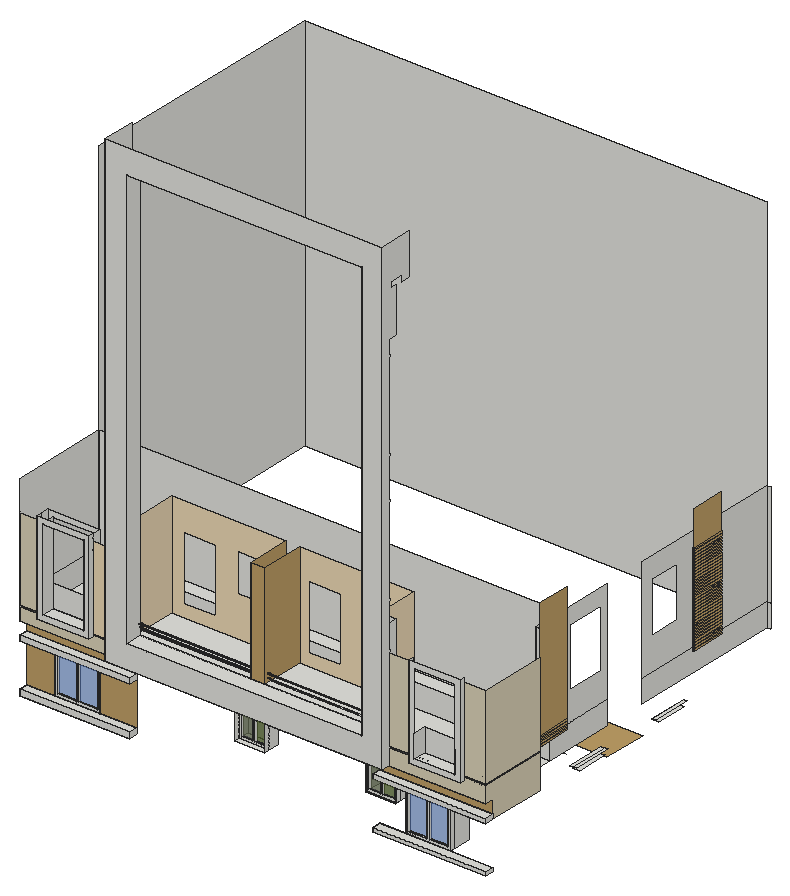
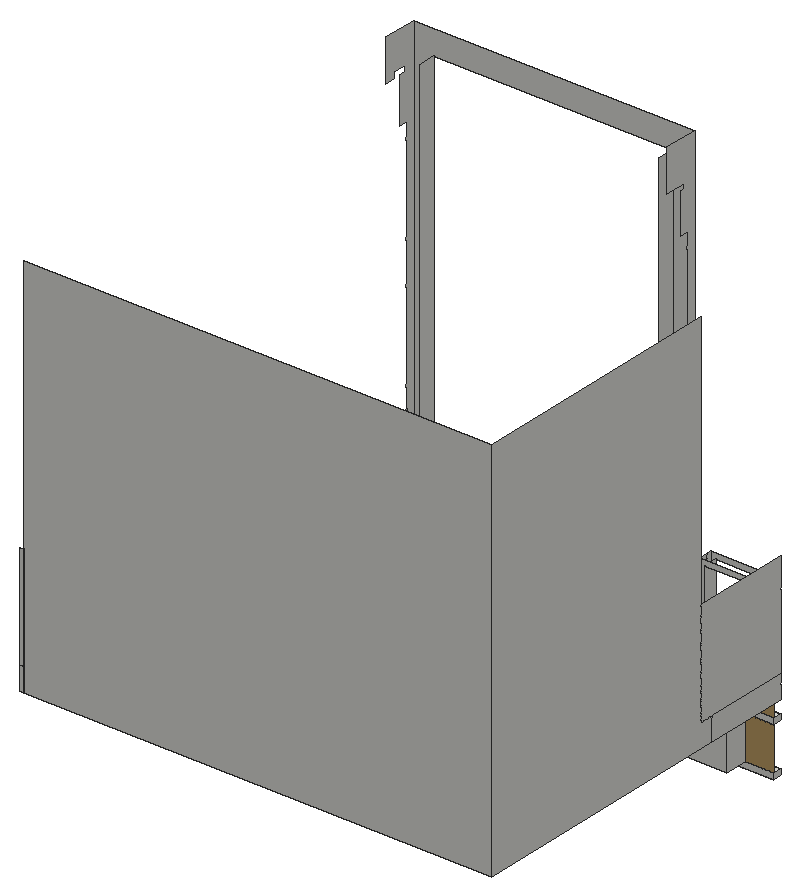
# SketchUp Ruby script. Lengths in inches.
U = 1.inch
M = Sketchup.active_model
def pt(a) = Geom::Point3d.new(a.map { |v| v * U })
def face(e, loops, mat)
  f = e.add_face(loops[0].map { |a| pt(a) })
  loops[1..].each { |l| e.add_face(l.map { |a| pt(a) }).erase! }
  f.material = f.back_material = mat if mat
  f
end
# faces: each face lists its corners as indices into pts; further lists are holes
def faces(e, pts, list, mat = nil) = list.each { |f| face(e, (f[0].is_a?(Array) ? f : [f]).map { |l| l.map { |i| pts[i] } }, mat) }
# xy, xz, yz: faces in a plane at the given z, y or x. An outline is a flat list of corners, or four numbers for a rectangle; further outlines are holes
def ring(l) = l.size == 4 ? [[l[0], l[1]], [l[2], l[1]], [l[2], l[3]], [l[0], l[3]]] : l.each_slice(2).to_a
def flat(e, list, mat, &to3) = list.each { |f| face(e, (f[0].is_a?(Array) ? f : [f]).map { |l| ring(l).map { |u, v| to3.(u, v) } }, mat) }
def xy(e, z, list, mat = nil) = flat(e, list, mat) { |x, y| [x, y, z] }
def xz(e, y, list, mat = nil) = flat(e, list, mat) { |x, z| [x, y, z] }
def yz(e, x, list, mat = nil) = flat(e, list, mat) { |y, z| [x, y, z] }
def lines(e, pts, list) = list.each { |a, b| e.add_line(pt(pts[a]), pt(pts[b])) }
# prism: a flat outline (further loops are holes) pulled along v
def prism(e, loops, v, mat = nil)
  f = face(e, loops, mat); d = Geom::Vector3d.new(v.map { |x| x * U })
  f.pushpull(f.normal.samedirection?(d) ? d.length : -d.length)
end
def box(e, o, s, mat = nil) = prism(e, [[o, [o[0] + s[0], o[1], o[2]], [o[0] + s[0], o[1] + s[1], o[2]], [o[0], o[1] + s[1], o[2]]]], [0, 0, s[2]], mat)
def at(x, y, z, deg = 0) = Geom::Transformation.translation(pt([x, y, z])) * Geom::Transformation.rotation(ORIGIN, Z_AXIS, deg.degrees)
def axes(o, x, y, z) = Geom::Transformation.new([*x, 0, *y, 0, *z, 0, *pt(o).to_a, 1])
def part(name) = M.definitions.add(name)
# library, detail: a bought-in or finely detailed component or shape, given as its bounding box
def library(name, o, s) = part(name).tap { |d| box(d.entities, o, s) }
def detail(e, o, s) = box(e.add_group.entities, o, s)
def put(e, d, t, mat = nil) = e.add_instance(d, t).tap { |i| i.material = mat if mat }
def group(e, t, mat = nil) = e.add_group.tap { |g| g.transformation = t; g.material = mat if mat }.entities
root = M.entities
M.materials.add("Generic").color = [191, 159, 103]
M.materials.add("Generic\#2").color = [235, 215, 180]
M.materials.add("Generic\#3").color = [218, 209, 183]
M.materials.add("[Color M06]").color = [86, 86, 86]
M.materials.add("[Translucent Glass Blue]").color = [100, 149, 237]
M.materials["[Translucent Glass Blue]"].alpha = 0.5
M.materials.add("[Translucent Glass Dark Green]").color = [62, 91, 5]
M.materials["[Translucent Glass Dark Green]"].alpha = 0.5
M.materials.add("[Translucent Glass Gray]").color = [128, 128, 128]
M.materials["[Translucent Glass Gray]"].alpha = 0.5
c1 = part("Group\#3")
xy(c1.entities,0,[[0,0,51.8125,6]])
xy(c1.entities,4.04,[[4.04,0,23.89,3],[27.93,0,47.77,3]])
xy(c1.entities,53.71,[[4.04,0,23.89,3],[27.93,0,47.77,3]])
xy(c1.entities,57.75,[[0,0,51.8125,6]])
xz(c1.entities,0,[[[0,0,51.8125,57.75],[4.04,4.04,23.89,53.71],[27.93,4.04,47.77,53.71]]])
xz(c1.entities,3,[[4.04,4.04,23.89,53.71],[27.93,4.04,47.77,53.71]],"[Translucent Glass Dark Green]")
xz(c1.entities,6,[[0,0,51.8125,57.75]],"[Translucent Glass Gray]")
yz(c1.entities,0,[[0,0,6,57.75]])
yz(c1.entities,4.04,[[0,4.04,3,53.71]])
yz(c1.entities,23.89,[[0,4.04,3,53.71]])
yz(c1.entities,27.93,[[0,4.04,3,53.71]])
yz(c1.entities,47.77,[[0,4.04,3,53.71]])
yz(c1.entities,51.8125,[[0,0,6,57.75]])
c2 = part("Group\#2")
xy(c2.entities,0,[[0,0,77.5625,6]])
xy(c2.entities,4.2,[[4.2,0,36.68,3],[40.88,0,73.36,3]])
xy(c2.entities,70.05,[[4.2,0,36.68,3],[40.88,0,73.36,3]])
xy(c2.entities,74.25,[[0,0,77.5625,6]])
xz(c2.entities,0,[[[0,0,77.5625,74.25],[40.88,4.2,73.36,70.05],[4.2,4.2,36.68,70.05]]])
xz(c2.entities,3,[[4.2,4.2,36.68,70.05],[40.88,4.2,73.36,70.05]],"[Translucent Glass Blue]")
xz(c2.entities,6,[[0,0,77.5625,74.25]])
yz(c2.entities,0,[[0,0,6,74.25]])
yz(c2.entities,4.2,[[0,4.2,3,70.05]])
yz(c2.entities,36.68,[[0,4.2,3,70.05]])
yz(c2.entities,40.88,[[0,4.2,3,70.05]])
yz(c2.entities,73.36,[[0,4.2,3,70.05]])
yz(c2.entities,77.5625,[[0,0,6,74.25]])
c3 = part("Group\#5")
xy(c3.entities,0,[[0,0,1,57.75]])
xy(c3.entities,2.57,[[0,0,1,57.75]])
xz(c3.entities,0,[[0,0,1,2.57]])
xz(c3.entities,57.75,[[0,0,1,2.57]])
yz(c3.entities,1,[[0,0,57.75,2.57]])
c4 = part("Group\#6")
put(c4.entities,c3,at(0,0,4.75))
put(c4.entities,c3,at(0,0,0))
put(c4.entities,c3,at(0,0,19))
put(c4.entities,c3,at(0,0,28.5))
put(c4.entities,c3,at(0,0,133))
put(c4.entities,c3,at(0,0,152))
put(c4.entities,c3,at(0,0,128.25))
put(c4.entities,c3,at(0,0,9.5))
put(c4.entities,c3,at(0,0,123.5))
put(c4.entities,c3,at(0,0,114))
put(c4.entities,c3,at(0,0,147.25))
put(c4.entities,c3,at(0,0,118.75))
put(c4.entities,c3,at(0,0,142.5))
put(c4.entities,c3,at(0,0,109.25))
put(c4.entities,c3,at(0,0,137.75))
put(c4.entities,c3,at(0,0,104.5))
put(c4.entities,c3,at(0,0,99.75))
put(c4.entities,c3,at(0,0,95))
put(c4.entities,c3,at(0,0,85.5))
put(c4.entities,c3,at(0,0,80.75))
put(c4.entities,c3,at(0,0,90.25))
put(c4.entities,c3,at(0,0,76))
put(c4.entities,c3,at(0,0,71.25))
put(c4.entities,c3,at(0,0,38))
put(c4.entities,c3,at(0,0,14.25))
put(c4.entities,c3,at(0,0,33.25))
put(c4.entities,c3,at(0,0,57))
put(c4.entities,c3,at(0,0,23.75))
put(c4.entities,c3,at(0,0,61.75))
put(c4.entities,c3,at(0,0,156.75))
put(c4.entities,c3,at(0,0,47.5))
put(c4.entities,c3,at(0,0,52.25))
put(c4.entities,c3,at(0,0,42.75))
put(c4.entities,c3,at(0,0,66.5))
xy(root,284.38,[[4.1875,68.4375,193.83,83.8125]])
xy(root,286.25,[[310.76,150.125,362.58,158.75],[536.08,150.125,587.89,158.75],[310.76,158.75,362.58,177.1875],[536.08,158.75,587.89,210.9375]])
xy(root,287.13,[[613.73,68.4375,809.375,83.8125]])
xy(root,294.19,[[4.1875,68.4375,193.83,83.8125],[613.73,68.4375,809.375,83.8125],[53.01,83.8125,130.57,121.875],[658.76,83.8125,736.32,121.875]])
xy(root,344,[[310.76,150.125,362.58,158.75],[536.08,150.125,587.89,158.75],[310.76,158.75,362.58,177.1875],[536.08,158.75,587.89,210.9375]])
xy(root,344.97,[[214.375,158.75,270.0625,214.75],[439.6875,158.75,495.375,214.75]])
xy(root,348.04,[[306.72,150.125,366.62,158.75],[532.04,150.125,591.93,158.75]])
xy(root,350.51,[[710.73,338.625,802.875,414.4375]],"Generic")
xy(root,367.13,[[802.875,263.64,815.3125,317.96],[802.875,434.88,815.3125,489.19]])
xy(root,368.44,[[4.1875,68.4375,193.83,83.8125],[53.01,83.8125,130.57,121.875],[658.76,83.8125,736.32,121.875]])
xy(root,368.76,[[613.23,68.4375,809.375,83.8125]])
xy(root,373.53,[[802.875,257.24,809.375,324.36],[809.375,257.24,815.3125,324.36],[809.375,428.47,815.3125,495.59]])
xy(root,376.76,[[613.23,68.4375,809.375,83.8125]])
xy(root,378.07,[[4.1875,68.4375,193.83,83.8125]])
xy(root,399.75,[[162.33,54.3125,641.55,83.8125],[4.1875,68.5,162.33,83.8125],[641.55,68.5,809.375,83.8125],[4.1875,83.8125,4.1875,214.75,802.875,214.75,802.875,83.8125,613.23,83.8125,613.23,158.75,415.53,158.75,415.53,83.8125,391.53,83.8125,391.53,158.75,193.83,158.75,193.83,83.8125],[193.83,83.8125,391.53,158.75],
  [415.53,83.8125,613.23,158.75]])
xy(root,419.29,[[40.68,60.5625,129.91,68.5],[40.68,68.5,129.91,83.8125]])
xy(root,421.51,[[4.1875,68.5,40.68,69.9375],[129.91,68.5,162.33,69.9375]])
xy(root,421.94,[[682.51,60.5625,771.75,68.5]])
xy(root,424.51,[[4.1875,68.5,40.68,69.9375],[129.91,68.5,162.33,69.9375]])
xy(root,427.125,[[641.55,68.5,682.51,69.9375],[771.75,68.5,802.875,69.9375],[802.875,68.5,809.375,69.9375],[807.9375,69.9375,809.375,185.01]])
xy(root,428.19,[[49.58,60.5625,121.01,83.8125]])
xy(root,430.125,[[641.55,68.5,682.51,69.9375],[771.75,68.5,809.375,69.9375],[807.9375,69.9375,809.375,185.01]])
xy(root,430.84,[[691.41,60.5625,762.85,83.8125]])
xy(root,439.5,[[200.02,54.3125,607.05,83.8125],[193.83,83.8125,391.53,158.75],[415.53,83.8125,613.23,158.75],[802.875,185.01,809.375,242.76],[4.1875,214.75,802.875,239.73]])
xz(root,54.3125,[[[162.33,399.75,641.55,1207.3125],[200.02,439.5,607.05,1165.125]]])
xz(root,60.5625,[[[40.68,419.29,129.91,578.68],[49.58,428.19,121.01,569.78]],[[682.51,421.94,771.75,581.34],[691.41,430.84,762.85,572.44]]])
xz(root,68.4375,[[4.1875,284.38,193.83,294.19],[613.73,287.13,809.375,294.19],[4.1875,368.44,193.83,378.07],[613.23,368.76,809.375,376.76]])
xz(root,68.5,[[129.35,421.51,129.91,424.51],[682.51,427.125,771.75,430.125]])
xz(root,68.5,[[129.91,424.51,162.33,567.15]],"Generic\#2")
xz(root,68.5,[[4.1875,399.75,162.33,399.75,162.33,421.51,129.91,421.51,129.91,419.29,40.68,419.29,40.68,421.51,4.1875,421.51],[641.55,399.75,809.375,399.75,809.375,427.125,771.75,427.125,771.75,421.94,682.51,421.94,682.51,427.125,641.55,427.125],[4.1875,424.51,40.68,567.15],[641.55,430.125,682.51,574.59],[771.75,430.125,809.375,574.59]],"Generic\#3")
xz(root,69.9375,[[4.1875,421.51,40.68,424.51],[129.91,421.51,162.33,424.51],[641.55,427.125,682.51,430.125],[771.75,427.125,807.9375,430.125]],"[Color M06]")
xz(root,83.8125,[[4.1875,284.38,193.83,294.19],[613.73,287.13,809.375,294.19],[4.1875,368.44,193.83,378.07],[613.23,368.76,809.375,376.76],[162.33,399.75,607.05,439.5],
  [607.05,399.75,641.55,439.5],[[40.68,419.29,129.91,578.68],[49.58,428.19,121.01,569.78]],[49.58,428.19,121.01,467.03],[691.41,430.84,762.85,469.69],[162.33,439.5,193.83,619.5],
  [193.83,439.5,200.02,619.5],[607.05,439.5,613.23,619.5],[613.23,439.5,641.55,619.5]])
xz(root,83.8125,[[4.1875,294.19,53.01,368.44],[130.57,294.19,193.83,368.44],[613.23,376.76,809.375,399.75],[4.1875,378.07,193.83,399.75],[391.53,439.5,415.53,619.5]],"Generic")
xz(root,121.875,[[53.01,294.19,130.57,368.44],[658.76,294.19,736.32,368.44]])
xz(root,158.75,[[[193.83,439.5,391.53,619.5],[215.38,461.3125,271.07,571.5625],[307.73,508.8,367.625,574.63]],[[415.53,439.5,613.23,619.5],[431.19,461.3125,486.88,571.5625],[523.54,508.8,583.4375,574.63]]],"Generic\#2")
xz(root,177.1875,[[310.76,286.25,362.58,344]])
xz(root,185.01,[[807.9375,427.125,809.375,430.125],[802.875,439.5,802.875,619.5,809.375,619.5,809.375,577.59,807.9375,577.59,807.9375,574.59,809.375,574.59,809.375,439.5]])
xz(root,210.9375,[[536.08,286.25,587.89,344]])
xz(root,214.75,[[4.1875,399.75,802.875,439.5]])
xz(root,239.73,[[4.1875,439.5,802.875,619.5]])
xz(root,242.76,[[802.875,439.5,809.375,619.5]])
xz(root,683.8125,[[4.1875,399.75,802.875,1059],[802.875,399.75,809.375,439.5],[802.875,439.5,809.375,619.5]])
yz(root,4.1875,[[68.4375,284.38,83.8125,294.19],[68.4375,368.44,83.8125,378.07],[68.5,399.75,68.5,421.51,69.9375,421.51,69.9375,424.51,68.5,424.51,68.5,439.5,214.75,439.5,214.75,399.75],[214.75,399.75,214.75,439.5,239.73,439.5,239.73,1059,683.8125,1059,683.8125,399.75],[68.5,439.5,68.5,567.15,69.9375,567.15,69.9375,570.15,68.5,570.15,68.5,619.5,239.73,619.5,239.73,439.5]])
yz(root,40.68,[[60.5625,419.29,68.5,419.29,68.5,421.51,69.9375,421.51,69.9375,424.51,68.5,424.51,68.5,567.15,69.9375,567.15,69.9375,570.15,68.5,570.15,68.5,578.68,60.5625,578.68],[68.5,419.29,83.8125,419.29,83.8125,578.68,68.5,578.68,68.5,570.15,69.9375,570.15,69.9375,567.15,68.5,567.15,68.5,424.51,69.9375,424.51,69.9375,421.51,68.5,421.51]])
yz(root,49.58,[[60.5625,428.19,83.8125,569.78]])
yz(root,53.01,[[83.8125,294.19,121.875,368.44]])
yz(root,121.01,[[60.5625,428.19,83.8125,569.78]])
yz(root,129.91,[[60.5625,419.29,68.5,578.68],[68.5,419.29,68.5,421.51,69.9375,421.51,69.9375,424.51,68.5,424.51,68.5,567.15,69.9375,567.15,69.9375,570.15,68.5,570.15,68.5,578.68,83.8125,578.68,83.8125,419.29],[68.5,421.51,69.9375,424.51]])
yz(root,130.57,[[83.8125,294.19,121.875,368.44]])
yz(root,162.33,[[54.3125,399.75,54.3125,1207.3125,112.625,1207.3125,112.625,1136.625,77.8125,1136.625,77.8125,1128.4375,83.8125,1128.4375,83.8125,1059,68.5,1059,68.5,1036.33,71.375,1036.33,71.375,1033.33,68.5,1033.33,68.5,882,69.9375,882,69.9375,879,68.5,879,68.5,806.75,69.9375,806.75,69.9375,803.75,68.5,803.75,68.5,658.14,69.9375,658.14,69.9375,655.14,68.5,655.14,68.5,570.15,69.9375,570.15,69.9375,567.15,68.5,567.15,68.5,424.51,69.9375,424.51,69.9375,421.51,68.5,421.51,68.5,399.75],[68.5,399.75,68.5,421.51,69.9375,421.51,69.9375,424.51,68.5,424.51,68.5,439.5,83.8125,439.5,83.8125,399.75],[68.5,439.5,68.5,567.15,69.9375,567.15,69.9375,570.15,68.5,570.15,68.5,619.5,83.8125,619.5,83.8125,439.5]])
yz(root,193.83,[[68.4375,284.38,83.8125,294.19],[68.4375,368.44,83.8125,378.07]])
yz(root,193.83,[[[83.8125,439.5,158.75,619.5],[90.04,472.27,89.73,472.3125,89.44,472.43,89.2,472.62,89.01,472.86,88.89,473.15,88.85,473.46,88.89,473.77,89.01,474.05,89.2,474.3,89.44,474.49,89.73,474.61,90.04,474.65,90.35,474.61,90.63,474.49,90.88,474.3,91.07,474.05,91.18,473.77,91.23,473.46,91.18,473.15,91.07,472.86,90.88,472.62,90.63,472.43,90.35,472.3125],[90.04,465.71,89.73,465.75,89.44,465.87,89.2,466.06,89.01,466.3,88.89,466.59,88.85,466.9,88.89,467.2,89.01,467.49,89.2,467.74,89.44,467.92,89.73,468.04,90.04,468.08,90.35,468.04,90.63,467.92,90.88,467.74,91.07,467.49,91.18,467.2,91.23,466.9,91.18,466.59,91.07,466.3,90.88,466.06,90.63,465.87,90.35,465.75],[90.04,458.71,89.73,458.75,89.44,458.87,89.2,459.06,89.01,459.3,88.89,459.59,88.85,459.9,88.89,460.2,89.01,460.49,89.2,460.74,89.44,460.92,89.73,461.04,90.04,461.08,90.35,461.04,90.63,460.92,90.88,460.74,91.07,460.49,91.18,460.2,91.23,459.9,91.18,459.59,91.07,459.3,90.88,459.06,90.63,458.87,90.35,458.75],[90.04,451.71,89.73,451.75,89.44,451.87,89.2,452.06,89.01,452.3,88.89,452.59,88.85,452.9,88.89,453.2,89.01,453.49,89.2,453.74,89.44,453.92,89.73,454.04,90.04,454.08,90.35,454.04,90.63,453.92,90.88,453.74,91.07,453.49,91.18,453.2,91.23,452.9,91.18,452.59,91.07,452.3,90.88,452.06,90.63,451.87,90.35,451.75],[90.04,445.02,89.73,445.0625,89.44,445.18,89.2,445.37,89.01,445.61,88.89,445.9,88.85,446.21,88.89,446.52,89.01,446.8,89.2,447.05,89.44,447.24,89.73,447.36,90.04,447.4,90.35,447.36,90.63,447.24,90.88,447.05,91.07,446.8,91.18,446.52,91.23,446.21,91.18,445.9,91.07,445.61,90.88,445.37,90.63,445.18,90.35,445.0625]]],"Generic\#2")
yz(root,200.02,[[54.3125,439.5,83.8125,1165.125]])
yz(root,310.76,[[150.125,286.25,158.75,344],[158.75,286.25,177.1875,344]])
yz(root,362.58,[[150.125,286.25,158.75,344],[158.75,286.25,177.1875,344]])
yz(root,391.53,[[[83.8125,439.5,158.75,619.5],[90.04,445.02,90.35,445.0625,90.63,445.18,90.88,445.37,91.07,445.61,91.18,445.9,91.23,446.21,91.18,446.52,91.07,446.8,90.88,447.05,90.63,447.24,90.35,447.36,90.04,447.4,89.73,447.36,89.44,447.24,89.2,447.05,89.01,446.8,88.89,446.52,88.85,446.21,88.89,445.9,89.01,445.61,89.2,445.37,89.44,445.18,89.73,445.0625],[90.04,451.71,90.35,451.75,90.63,451.87,90.88,452.06,91.07,452.3,91.18,452.59,91.23,452.9,91.18,453.2,91.07,453.49,90.88,453.74,90.63,453.92,90.35,454.04,90.04,454.08,89.73,454.04,89.44,453.92,89.2,453.74,89.01,453.49,88.89,453.2,88.85,452.9,88.89,452.59,89.01,452.3,89.2,452.06,89.44,451.87,89.73,451.75],[90.04,458.71,90.35,458.75,90.63,458.87,90.88,459.06,91.07,459.3,91.18,459.59,91.23,459.9,91.18,460.2,91.07,460.49,90.88,460.74,90.63,460.92,90.35,461.04,90.04,461.08,89.73,461.04,89.44,460.92,89.2,460.74,89.01,460.49,88.89,460.2,88.85,459.9,88.89,459.59,89.01,459.3,89.2,459.06,89.44,458.87,89.73,458.75],[90.04,465.71,90.35,465.75,90.63,465.87,90.88,466.06,91.07,466.3,91.18,466.59,91.23,466.9,91.18,467.2,91.07,467.49,90.88,467.74,90.63,467.92,90.35,468.04,90.04,468.08,89.73,468.04,89.44,467.92,89.2,467.74,89.01,467.49,88.89,467.2,88.85,466.9,88.89,466.59,89.01,466.3,89.2,466.06,89.44,465.87,89.73,465.75],[90.04,472.27,90.35,472.3125,90.63,472.43,90.88,472.62,91.07,472.86,91.18,473.15,91.23,473.46,91.18,473.77,91.07,474.05,90.88,474.3,90.63,474.49,90.35,474.61,90.04,474.65,89.73,474.61,89.44,474.49,89.2,474.3,89.01,474.05,88.89,473.77,88.85,473.46,88.89,473.15,89.01,472.86,89.2,472.62,89.44,472.43,89.73,472.3125]]],"Generic")
yz(root,415.53,[[[83.8125,439.5,158.75,619.5],[89.21,476.09,89.0625,476.11,88.93,476.16,88.8125,476.25,88.72,476.37,88.67,476.5,88.65,476.65,88.67,476.79,88.72,476.93,88.8125,477.05,88.93,477.14,89.0625,477.19,89.21,477.21,89.36,477.19,89.49,477.14,89.61,477.05,89.7,476.93,89.75,476.79,89.77,476.65,89.75,476.5,89.7,476.37,89.61,476.25,89.49,476.16,89.36,476.11],[89.21,468.65,89.0625,468.67,88.93,468.72,88.8125,468.8125,88.72,468.93,88.67,469.07,88.65,469.21,88.67,469.36,88.72,469.49,88.8125,469.61,88.93,469.7,89.0625,469.76,89.21,469.77,89.36,469.76,89.49,469.7,89.61,469.61,89.7,469.49,89.75,469.36,89.77,469.21,89.75,469.07,89.7,468.93,89.61,468.8125,89.49,468.72,89.36,468.67],[89.21,461.15,89.0625,461.17,88.93,461.22,88.8125,461.3125,88.72,461.43,88.67,461.57,88.65,461.71,88.67,461.86,88.72,461.99,88.8125,462.11,88.93,462.2,89.0625,462.26,89.21,462.27,89.36,462.26,89.49,462.2,89.61,462.11,89.7,461.99,89.75,461.86,89.77,461.71,89.75,461.57,89.7,461.43,89.61,461.3125,89.49,461.22,89.36,461.17],[89.21,453.65,89.0625,453.67,88.93,453.72,88.8125,453.8125,88.72,453.93,88.67,454.07,88.65,454.21,88.67,454.36,88.72,454.49,88.8125,454.61,88.93,454.7,89.0625,454.76,89.21,454.77,89.36,454.76,89.49,454.7,89.61,454.61,89.7,454.49,89.75,454.36,89.77,454.21,89.75,454.07,89.7,453.93,89.61,453.8125,89.49,453.72,89.36,453.67],[89.21,446.27,89.0625,446.29,88.93,446.35,88.8125,446.4375,88.72,446.56,88.67,446.69,88.65,446.84,88.67,446.98,88.72,447.12,88.8125,447.23,88.93,447.32,89.0625,447.38,89.21,447.4,89.36,447.38,89.49,447.32,89.61,447.23,89.7,447.12,89.75,446.98,89.77,446.84,89.75,446.69,89.7,446.56,89.61,446.4375,89.49,446.35,89.36,446.29]]],"Generic")
yz(root,536.08,[[150.125,286.25,158.75,344],[158.75,286.25,210.9375,344]])
yz(root,587.89,[[150.125,286.25,158.75,344],[158.75,286.25,210.9375,344]])
yz(root,607.05,[[54.3125,439.5,83.8125,1165.125]])
yz(root,613.23,[[68.4375,368.76,83.8125,376.76]])
yz(root,613.23,[[[83.8125,439.5,158.75,619.5],[89.21,446.27,89.36,446.29,89.49,446.35,89.61,446.4375,89.7,446.56,89.75,446.69,89.77,446.84,89.75,446.98,89.7,447.12,89.61,447.23,89.49,447.32,89.36,447.38,89.21,447.4,89.0625,447.38,88.93,447.32,88.8125,447.23,88.72,447.12,88.67,446.98,88.65,446.84,88.67,446.69,88.72,446.56,88.8125,446.4375,88.93,446.35,89.0625,446.29],[89.21,453.65,89.36,453.67,89.49,453.72,89.61,453.8125,89.7,453.93,89.75,454.07,89.77,454.21,89.75,454.36,89.7,454.49,89.61,454.61,89.49,454.7,89.36,454.76,89.21,454.77,89.0625,454.76,88.93,454.7,88.8125,454.61,88.72,454.49,88.67,454.36,88.65,454.21,88.67,454.07,88.72,453.93,88.8125,453.8125,88.93,453.72,89.0625,453.67],[89.21,461.15,89.36,461.17,89.49,461.22,89.61,461.3125,89.7,461.43,89.75,461.57,89.77,461.71,89.75,461.86,89.7,461.99,89.61,462.11,89.49,462.2,89.36,462.26,89.21,462.27,89.0625,462.26,88.93,462.2,88.8125,462.11,88.72,461.99,88.67,461.86,88.65,461.71,88.67,461.57,88.72,461.43,88.8125,461.3125,88.93,461.22,89.0625,461.17],[89.21,468.65,89.36,468.67,89.49,468.72,89.61,468.8125,89.7,468.93,89.75,469.07,89.77,469.21,89.75,469.36,89.7,469.49,89.61,469.61,89.49,469.7,89.36,469.76,89.21,469.77,89.0625,469.76,88.93,469.7,88.8125,469.61,88.72,469.49,88.67,469.36,88.65,469.21,88.67,469.07,88.72,468.93,88.8125,468.8125,88.93,468.72,89.0625,468.67],[89.21,476.09,89.36,476.11,89.49,476.16,89.61,476.25,89.7,476.37,89.75,476.5,89.77,476.65,89.75,476.79,89.7,476.93,89.61,477.05,89.49,477.14,89.36,477.19,89.21,477.21,89.0625,477.19,88.93,477.14,88.8125,477.05,88.72,476.93,88.67,476.79,88.65,476.65,88.67,476.5,88.72,476.37,88.8125,476.25,88.93,476.16,89.0625,476.11]]],"Generic\#2")
yz(root,613.73,[[68.4375,287.13,83.8125,294.19]])
yz(root,641.55,[[54.3125,399.75,68.5,399.75,68.5,427.125,69.9375,427.125,69.9375,430.125,68.5,430.125,68.5,574.59,69.9375,574.59,69.9375,577.59,68.5,577.59,68.5,653.5625,69.9375,653.5625,69.9375,656.5625,68.5,656.5625,68.5,806.5,69.9375,806.5,69.9375,809.5,68.5,809.5,68.5,879,69.9375,879,69.9375,882,68.5,882,68.5,1031.12,69.9375,1031.12,69.9375,1034.12,68.5,1034.12,68.5,1059,83.8125,1059,83.8125,1136.625,73.875,1136.625,73.875,1146.5625,95.8125,1146.5625,95.8125,1136.625,112.625,1136.625,112.625,1207.3125,54.3125,1207.3125],[68.5,399.75,83.8125,399.75,83.8125,439.5,68.5,439.5,68.5,430.125,69.9375,430.125,69.9375,427.125,68.5,427.125],[68.5,439.5,83.8125,439.5,83.8125,619.5,68.5,619.5,68.5,577.59,69.9375,577.59,69.9375,574.59,68.5,574.59]])
yz(root,658.76,[[83.8125,294.19,121.875,368.44]])
yz(root,682.51,[[60.5625,421.94,68.5,581.34],[68.5,427.125,69.9375,430.125]])
yz(root,691.41,[[60.5625,430.84,83.8125,469.69]])
yz(root,736.32,[[83.8125,294.19,121.875,368.44]])
yz(root,762.85,[[60.5625,430.84,83.8125,469.69]])
yz(root,771.75,[[60.5625,421.94,68.5,581.34],[68.5,427.125,69.9375,430.125]])
yz(root,802.875,[[214.75,399.75,338.625,439.5],[413.6875,399.75,683.8125,439.5],[185.01,439.5,239.73,619.5],[239.73,439.5,242.76,619.5],[[242.76,439.5,338.625,619.5],[257.24,489.97,324.36,590.66]],
  [[413.6875,439.5,683.8125,619.5],[434.88,496.375,489.19,584.25]]])
yz(root,807.9375,[[69.9375,427.125,185.01,430.125]],"[Color M06]")
yz(root,809.375,[[68.4375,287.13,83.8125,294.19],[68.4375,368.76,83.8125,376.76]])
yz(root,809.375,[[185.01,439.5,242.76,659.25],[518.09,439.5,575.84,659.25]],"Generic")
yz(root,809.375,[[83.8125,368.76,185.01,368.76,185.01,427.125,68.5,427.125,68.5,399.75,83.8125,399.75],[68.5,430.125,185.01,574.59]],"Generic\#3")
p = [[193.83,89.73,445.0625],[193.83,90.04,445.02],[391.53,90.04,445.02],[391.53,89.73,445.0625],[193.83,90.35,445.0625],[391.53,90.35,445.0625],
  [193.83,89.44,445.18],[391.53,89.44,445.18],[193.83,90.63,445.18],[391.53,90.63,445.18],[193.83,89.2,445.37],[391.53,89.2,445.37],
  [193.83,90.88,445.37],[391.53,90.88,445.37],[193.83,89.01,445.61],[391.53,89.01,445.61],[193.83,91.07,445.61],[391.53,91.07,445.61],
  [193.83,88.89,445.9],[391.53,88.89,445.9],[193.83,91.18,445.9],[391.53,91.18,445.9],[193.83,88.85,446.21],[391.53,88.85,446.21],
  [193.83,91.23,446.21],[391.53,91.23,446.21],[193.83,88.89,446.52],[391.53,88.89,446.52],[193.83,91.18,446.52],[391.53,91.18,446.52],
  [415.53,88.8125,446.4375],[415.53,88.93,446.35],[613.23,88.93,446.35],[613.23,88.8125,446.4375],[415.53,89.0625,446.29],[613.23,89.0625,446.29],
  [415.53,89.21,446.27],[613.23,89.21,446.27],[415.53,89.36,446.29],[613.23,89.36,446.29],[415.53,89.49,446.35],[613.23,89.49,446.35],
  [415.53,89.61,446.4375],[613.23,89.61,446.4375],[415.53,88.72,446.56],[613.23,88.72,446.56],[415.53,89.7,446.56],[613.23,89.7,446.56],
  [193.83,89.01,446.8],[391.53,89.01,446.8],[193.83,91.07,446.8],[391.53,91.07,446.8],[415.53,88.67,446.69],[613.23,88.67,446.69],
  [415.53,89.75,446.69],[613.23,89.75,446.69],[415.53,88.65,446.84],[613.23,88.65,446.84],[415.53,89.77,446.84],[613.23,89.77,446.84],
  [415.53,88.67,446.98],[613.23,88.67,446.98],[193.83,89.2,447.05],[391.53,89.2,447.05],[415.53,89.75,446.98],[613.23,89.75,446.98],
  [193.83,90.88,447.05],[391.53,90.88,447.05],[415.53,88.72,447.12],[613.23,88.72,447.12],[193.83,89.44,447.24],[391.53,89.44,447.24],
  [415.53,89.7,447.12],[613.23,89.7,447.12],[193.83,90.63,447.24],[391.53,90.63,447.24],[415.53,88.8125,447.23],[613.23,88.8125,447.23],
  [415.53,89.61,447.23],[613.23,89.61,447.23],[415.53,88.93,447.32],[613.23,88.93,447.32],[193.83,89.73,447.36],[391.53,89.73,447.36],
  [415.53,89.49,447.32],[613.23,89.49,447.32],[193.83,90.35,447.36],[391.53,90.35,447.36],[415.53,89.0625,447.38],[613.23,89.0625,447.38],
  [415.53,89.36,447.38],[613.23,89.36,447.38],[415.53,89.21,447.4],[613.23,89.21,447.4],[193.83,90.04,447.4],[391.53,90.04,447.4],
  [193.83,89.44,451.87],[193.83,89.73,451.75],[391.53,89.73,451.75],[391.53,89.44,451.87],[193.83,90.04,451.71],[391.53,90.04,451.71],
  [193.83,90.35,451.75],[391.53,90.35,451.75],[193.83,90.63,451.87],[391.53,90.63,451.87],[193.83,89.2,452.06],[391.53,89.2,452.06],
  [193.83,90.88,452.06],[391.53,90.88,452.06],[193.83,89.01,452.3],[391.53,89.01,452.3],[193.83,91.07,452.3],[391.53,91.07,452.3],
  [193.83,88.89,452.59],[391.53,88.89,452.59],[193.83,91.18,452.59],[391.53,91.18,452.59],[193.83,88.85,452.9],[391.53,88.85,452.9],
  [193.83,91.23,452.9],[391.53,91.23,452.9],[193.83,88.89,453.2],[391.53,88.89,453.2],[193.83,91.18,453.2],[391.53,91.18,453.2],
  [193.83,89.01,453.49],[391.53,89.01,453.49],[193.83,91.07,453.49],[391.53,91.07,453.49],[193.83,89.2,453.74],[391.53,89.2,453.74],
  [193.83,90.88,453.74],[391.53,90.88,453.74],[415.53,89.0625,453.67],[415.53,89.21,453.65],[613.23,89.21,453.65],[613.23,89.0625,453.67],
  [415.53,89.36,453.67],[613.23,89.36,453.67],[415.53,88.8125,453.8125],[415.53,88.93,453.72],[613.23,88.93,453.72],[613.23,88.8125,453.8125],
  [193.83,89.44,453.92],[391.53,89.44,453.92],[415.53,89.49,453.72],[613.23,89.49,453.72],[415.53,89.61,453.8125],[613.23,89.61,453.8125],
  [193.83,90.63,453.92],[391.53,90.63,453.92],[415.53,88.72,453.93],[613.23,88.72,453.93],[415.53,89.7,453.93],[613.23,89.7,453.93],
  [415.53,88.67,454.07],[613.23,88.67,454.07],[193.83,89.73,454.04],[391.53,89.73,454.04],[415.53,89.75,454.07],[613.23,89.75,454.07],
  [193.83,90.35,454.04],[391.53,90.35,454.04],[193.83,90.04,454.08],[391.53,90.04,454.08],[415.53,88.65,454.21],[613.23,88.65,454.21],
  [415.53,89.77,454.21],[613.23,89.77,454.21],[415.53,88.67,454.36],[613.23,88.67,454.36],[415.53,89.75,454.36],[613.23,89.75,454.36],
  [415.53,88.72,454.49],[613.23,88.72,454.49],[415.53,89.7,454.49],[613.23,89.7,454.49],[415.53,88.8125,454.61],[613.23,88.8125,454.61],
  [415.53,89.61,454.61],[613.23,89.61,454.61],[415.53,88.93,454.7],[613.23,88.93,454.7],[415.53,89.49,454.7],[613.23,89.49,454.7],
  [415.53,89.0625,454.76],[613.23,89.0625,454.76],[415.53,89.36,454.76],[613.23,89.36,454.76],[415.53,89.21,454.77],[613.23,89.21,454.77],
  [802.875,68.5,439.5],[802.875,185.01,439.5],[415.53,95.8125,439.5],[607.05,95.8125,439.5],[415.53,89.21,446.93],[613.23,89.21,446.93],
  [415.53,89.21,454.37],[613.23,89.21,454.37],[193.83,90.04,446.27],[391.53,90.04,446.27],[193.83,90.04,453.02],[391.53,90.04,453.02],
  [802.875,242.76,399.75],[809.375,242.76,399.75]]
faces(root,p,[[0,1,2,3],[1,4,5,2],[6,0,3,7],[4,8,9,5],[10,6,7,11],[8,12,13,9],[14,10,11,15],[12,16,17,13],
  [18,14,15,19],[16,20,21,17],[22,18,19,23],[20,24,25,21],[26,22,23,27],[24,28,29,25],[30,31,32,33],[31,34,35,32],
  [34,36,37,35],[36,38,39,37],[38,40,41,39],[40,42,43,41],[44,30,33,45],[42,46,47,43],[48,26,27,49],[28,50,51,29],
  [52,44,45,53],[46,54,55,47],[56,52,53,57],[54,58,59,55],[60,56,57,61],[62,48,49,63],[58,64,65,59],[50,66,67,51],
  [68,60,61,69],[70,62,63,71],[64,72,73,65],[66,74,75,67],[76,68,69,77],[72,78,79,73],[80,76,77,81],[82,70,71,83],
  [78,84,85,79],[74,86,87,75],[88,80,81,89],[84,90,91,85],[92,88,89,93],[90,92,93,91],[94,82,83,95],[86,94,95,87],
  [96,97,98,99],[97,100,101,98],[100,102,103,101],[102,104,105,103],[106,96,99,107],[104,108,109,105],[110,106,107,111],[108,112,113,109],
  [114,110,111,115],[112,116,117,113],[118,114,115,119],[116,120,121,117],[122,118,119,123],[120,124,125,121],[126,122,123,127],[124,128,129,125],
  [130,126,127,131],[128,132,133,129],[134,135,136,137],[135,138,139,136],[140,141,142,143],[141,134,137,142],[144,130,131,145],[138,146,147,139],
  [146,148,149,147],[132,150,151,133],[152,140,143,153],[148,154,155,149],[156,152,153,157],[158,144,145,159],[154,160,161,155],[150,162,163,151],
  [164,158,159,165],[162,164,165,163],[166,156,157,167],[160,168,169,161],[170,166,167,171],[168,172,173,169],[174,170,171,175],[172,176,177,173],
  [178,174,175,179],[176,180,181,177],[182,178,179,183],[180,184,185,181],[186,182,183,187],[184,188,189,185],[190,186,187,191],[188,190,191,189]])
lines(root,p,[[192,193],[194,195],[196,197],[198,199],[200,201],[202,203],[204,205]])
put(root,c1,at(310.76,158.75,286.25))
put(root,c1,at(536.08,152.75,286.25))
put(root,c2,at(53.01,83.8125,294.19))
put(root,c2,at(658.76,83.8125,294.19))
put(root,c3,at(809.375,185.01,437.33),"Generic")
put(root,c4,at(807.375,518.09,437.86))
put(root,c4,at(809.375,518.09,439.5),"Generic")
put(root,c3,at(809.375,185.01,442.08),"Generic")
put(root,c3,at(809.375,185.01,446.83),"Generic")
put(root,c3,at(809.375,185.01,451.58),"Generic")
